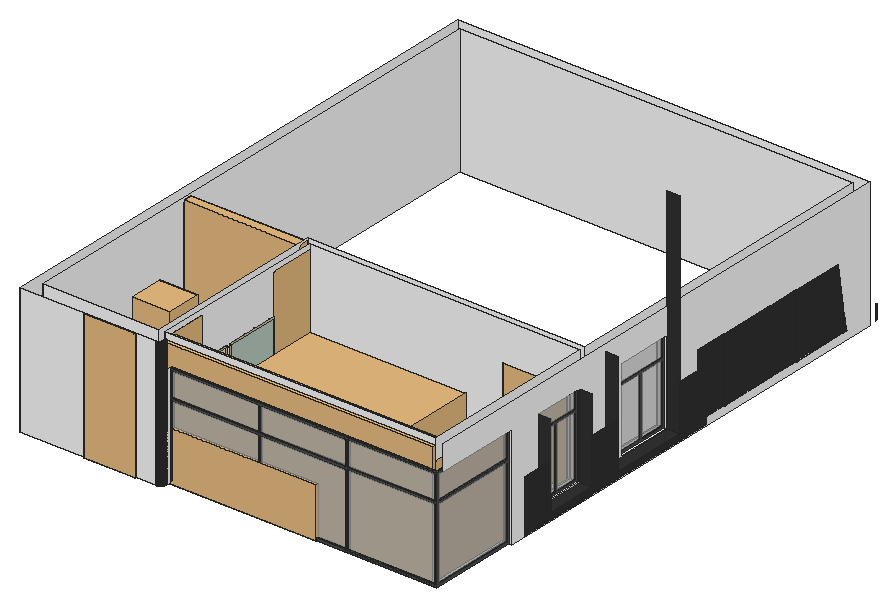
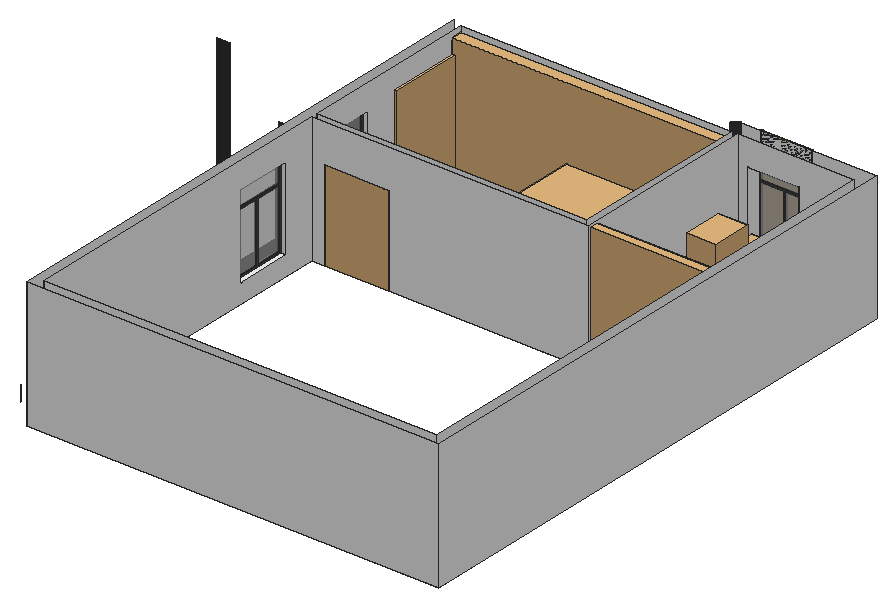
# SketchUp Ruby script. Lengths in inches.
U = 1.inch
M = Sketchup.active_model
def pt(a) = Geom::Point3d.new(a.map { |v| v * U })
def face(e, loops, mat)
  f = e.add_face(loops[0].map { |a| pt(a) })
  loops[1..].each { |l| e.add_face(l.map { |a| pt(a) }).erase! }
  f.material = f.back_material = mat if mat
  f
end
# faces: each face lists its corners as indices into pts; further lists are holes
def faces(e, pts, list, mat = nil) = list.each { |f| face(e, (f[0].is_a?(Array) ? f : [f]).map { |l| l.map { |i| pts[i] } }, mat) }
# xy, xz, yz: faces in a plane at the given z, y or x. An outline is a flat list of corners, or four numbers for a rectangle; further outlines are holes
def ring(l) = l.size == 4 ? [[l[0], l[1]], [l[2], l[1]], [l[2], l[3]], [l[0], l[3]]] : l.each_slice(2).to_a
def flat(e, list, mat, &to3) = list.each { |f| face(e, (f[0].is_a?(Array) ? f : [f]).map { |l| ring(l).map { |u, v| to3.(u, v) } }, mat) }
def xy(e, z, list, mat = nil) = flat(e, list, mat) { |x, y| [x, y, z] }
def xz(e, y, list, mat = nil) = flat(e, list, mat) { |x, z| [x, y, z] }
def yz(e, x, list, mat = nil) = flat(e, list, mat) { |y, z| [x, y, z] }
def lines(e, pts, list) = list.each { |a, b| e.add_line(pt(pts[a]), pt(pts[b])) }
# prism: a flat outline (further loops are holes) pulled along v
def prism(e, loops, v, mat = nil)
  f = face(e, loops, mat); d = Geom::Vector3d.new(v.map { |x| x * U })
  f.pushpull(f.normal.samedirection?(d) ? d.length : -d.length)
end
def box(e, o, s, mat = nil) = prism(e, [[o, [o[0] + s[0], o[1], o[2]], [o[0] + s[0], o[1] + s[1], o[2]], [o[0], o[1] + s[1], o[2]]]], [0, 0, s[2]], mat)
def at(x, y, z, deg = 0) = Geom::Transformation.translation(pt([x, y, z])) * Geom::Transformation.rotation(ORIGIN, Z_AXIS, deg.degrees)
def axes(o, x, y, z) = Geom::Transformation.new([*x, 0, *y, 0, *z, 0, *pt(o).to_a, 1])
def part(name) = M.definitions.add(name)
# library, detail: a bought-in or finely detailed component or shape, given as its bounding box
def library(name, o, s) = part(name).tap { |d| box(d.entities, o, s) }
def detail(e, o, s) = box(e.add_group.entities, o, s)
def put(e, d, t, mat = nil) = e.add_instance(d, t).tap { |i| i.material = mat if mat }
def group(e, t, mat = nil) = e.add_group.tap { |g| g.transformation = t; g.material = mat if mat }.entities
root = M.entities
M.materials.add("12_plywood texture-seamless").color = [215, 194, 159]
M.materials.add("[Color_001]2").color = [144, 137, 126]
M.materials.add("[Color_005]1").color = [178, 182, 175]
M.materials.add("[Granite Dark Gray]").color = [51, 50, 50]
M.materials.add("[Metal Seamed]").color = [79, 80, 77]
M.materials.add("[Quartz Light Grey]").color = [251, 251, 252]
M.materials.add("[Translucent Glass Gray]").color = [183, 183, 183]
M.materials["[Translucent Glass Gray]"].alpha = 0.5
M.materials.add("[Wood Veneer 01]1").color = [120, 70, 37]
M.materials.add("il_570xN.1307621332_kpxq").color = [189, 207, 195]
M.materials.add("il_570xN.1571116333_4k0l").color = [234, 234, 226]
c1 = library("plant\#1",[-21.34,-27.21,-0.38],[41.91,41.15,38.97])
c2 = library("Classic grayblue sofa  living room ",[-100.93,-81.02,-0.06],[174.43,145.32,46.54])
c3 = library("small sofa",[87.94,-13.34,0],[66.53,49.05,32.95])
c4 = part("6\#1")
g1 = group(c4.entities,at(25.4,42.84,0),"[Color_001]2")
box(g1,[0,0,0],[104,190.3125,0.89],"[Color_005]1")
c5 = library("Plante 4",[-1.67,-6.5,0],[37.31,31.95,64.42])
c6 = library("Group\#15",[0,-0.5,0],[48,0.5,120])
c7 = part("Group\#22")
box(c7.entities,[0,-0.47,69],[80.67,0.47,23])
box(c7.entities,[0,-0.47,0],[80.67,0.47,67])
c8 = library("Group\#62",[0,0,0],[0.25,42,120])
c9 = library("Group\#68",[0,0,0],[0.25,42,120])
c10 = library("SLIDING+GLASS+DOOR",[0,-0.75,0],[72,5.75,80])
c11 = library("Curtains and rod",[2.63,-1.46,0.02],[153.32,14.02,114.15])
c12 = library("Curtains",[0,0,0],[121.73,8.19,117.22])
c13 = library("---------1\#1",[5.49,6.625,-77.21],[69.81,13.39,114.05])
c14 = part("Agrupar\#2")
xy(c14.entities,0,[[0,0,15.75,21.65]])
xy(c14.entities,0.59,[[0,0,15.75,21.65]],"il_570xN.1571116333_4k0l")
xz(c14.entities,0,[[0,0,15.75,0.59]])
xz(c14.entities,21.65,[[0,0,15.75,0.59]])
yz(c14.entities,0,[[0,0,21.65,0.59]])
yz(c14.entities,15.75,[[0,0,21.65,0.59]])
c15 = part("Agrupar\#4")
xy(c15.entities,0,[[[0.3,0.3,17.03,22.93],[0.79,0.79,16.54,22.44]]],"12_plywood texture-seamless")
xy(c15.entities,0.79,[[0.3,0.3,0.79,0.79,0.79,22.44,0.3,22.93],[0.3,0.3,17.03,0.3,16.54,0.79,0.79,0.79],[17.03,0.3,17.03,22.93,16.54,22.44,16.54,0.79],[0.79,22.44,16.54,22.44,17.03,22.93,0.3,22.93]],"12_plywood texture-seamless")
xz(c15.entities,0.3,[[0.3,0,17.03,0.79]],"12_plywood texture-seamless")
xz(c15.entities,0.79,[[0.79,0,16.54,0.79]],"12_plywood texture-seamless")
xz(c15.entities,22.44,[[0.79,0,16.54,0.79]],"12_plywood texture-seamless")
xz(c15.entities,22.93,[[0.3,0,17.03,0.79]],"12_plywood texture-seamless")
yz(c15.entities,0.3,[[0.3,0,22.93,0.79]],"12_plywood texture-seamless")
yz(c15.entities,0.79,[[0.79,0,22.44,0.79]],"12_plywood texture-seamless")
yz(c15.entities,16.54,[[0.79,0,22.44,0.79]],"12_plywood texture-seamless")
yz(c15.entities,17.03,[[0.3,0,22.93,0.79]],"12_plywood texture-seamless")
c16 = part("Agrupar\#1")
put(c16.entities,c14,at(0.79,0.79,0))
put(c16.entities,c15,at(0,0,0))
c17 = part("Agrupar\#3")
xy(c17.entities,0,[[-3.44,0,15.75,26.08]])
xy(c17.entities,0.59,[[-3.44,0,15.75,26.08]],"il_570xN.1307621332_kpxq")
xz(c17.entities,0,[[-3.44,0,15.75,0.59]])
xz(c17.entities,26.08,[[-3.44,0,15.75,0.59]])
yz(c17.entities,-3.44,[[0,0,26.08,0.59]])
yz(c17.entities,15.75,[[0,0,26.08,0.59]])
c18 = part("Agrupar\#7")
xy(c18.entities,0,[[[-3.15,0.3,17.03,27.36],[-2.66,0.79,16.54,26.87]]],"12_plywood texture-seamless")
xy(c18.entities,0.79,[[-3.15,0.3,-3.15,27.36,-2.66,26.87,-2.66,0.79],[-3.15,0.3,17.03,0.3,16.54,0.79,-2.66,0.79],[17.03,0.3,16.54,0.79,16.54,26.87,17.03,27.36],[-2.66,26.87,-3.15,27.36,17.03,27.36,16.54,26.87]],"12_plywood texture-seamless")
xz(c18.entities,0.3,[[-3.15,0,17.03,0.79]],"12_plywood texture-seamless")
xz(c18.entities,0.79,[[-2.66,0,16.54,0.79]],"12_plywood texture-seamless")
xz(c18.entities,26.87,[[-2.66,0,16.54,0.79]],"12_plywood texture-seamless")
xz(c18.entities,27.36,[[-3.15,0,17.03,0.79]],"12_plywood texture-seamless")
yz(c18.entities,-3.15,[[0.3,0,27.36,0.79]],"12_plywood texture-seamless")
yz(c18.entities,-2.66,[[0.79,0,26.87,0.79]],"12_plywood texture-seamless")
yz(c18.entities,16.54,[[0.79,0,26.87,0.79]],"12_plywood texture-seamless")
yz(c18.entities,17.03,[[0.3,0,27.36,0.79]],"12_plywood texture-seamless")
c19 = part("Agrupar\#8")
put(c19.entities,c17,at(0.79,0.79,0))
put(c19.entities,c18,at(0,0,0))
c20 = part("CALIFORNIA WALL ART")
put(c20.entities,c16,axes([-38.21,13.68,-7.42],[0.78256,0,0],[0,0,0.78256],[0,-0.78256,0]))
put(c20.entities,c19,axes([-23.17,13.75,7.77],[0,0,-0.878],[0.878,0,0],[0,-0.878,0]))
xy(root,138,[[48,90,48,600,432,600,432,183,423,183,423,591,57,591,57,105,165,105,165,279,351,279,351,273,171,273,171,105,180,105,180,95.78,179.95,95.23,179.93,95.12,179.92,95.01,179.9,94.9,179.85,94.68,179.83,94.57,179.8,94.46,179.77,94.36,179.74,94.25,179.71,94.15,179.67,94.04,179.63,93.9375,179.59,93.83,179.47,93.53,179.27,93.13,179.21,93.03,179.16,92.9375,179.1,92.84,178.98,92.66,178.92,92.5625,178.85,92.47,178.79,92.38,178.72,92.3,178.65,92.21,178.51,92.04,178.43,91.96,178.36,91.875,178.28,91.8,178.2,91.72,178.125,91.64,178.04,91.57,177.96,91.49,177.79,91.35,177.7,91.28,177.62,91.21,177.53,91.15,177.4375,91.08,177.34,91.02,177.16,90.9,177.0625,90.84,176.97,90.79,176.87,90.73,176.47,90.53,176.17,90.41,176.0625,90.37,175.96,90.33,175.85,90.29,175.75,90.26,175.64,90.23,175.54,90.2,175.43,90.17,175.32,90.15,175.1,90.1,174.99,90.08,174.88,90.07,174.77,90.05,174.22,90],[411,273,423,279]],"[Quartz Light Grey]")
xy(root,150,[[443.875,183,444,207],[443.875,208,444,213],[443.875,213,444,261],[443.875,261,444,267],[443.875,268,444,291],
  [443.875,291,444,303],[443.875,304,444,369],[443.875,370,444,393],[436.875,393,437,423],[436.875,424,437,477],
  [436.875,478,437,507],[436.875,508,437,562],[436.875,563,437,565.83]],"[Granite Dark Gray]")
xy(root,151,[[443.875,183,444,207],[443.875,208,444,213],[443.875,213,444,261],[443.875,261,444,267],[443.875,268,444,291],
  [443.875,291,444,369],[443.875,370,444,393],[436.875,393,437,423],[436.875,424,437,477],[436.875,478,437,507],
  [436.875,508,437,562],[436.875,563,437,565.65]],"[Granite Dark Gray]")
xy(root,156,[[432,213,444,261],[432,291,444,363]],"[Granite Dark Gray]")
xy(root,156,[[423,213,432,261],[423,309,432,363]],"[Quartz Light Grey]")
xy(root,162,[[108,90,156,105]],"[Quartz Light Grey]")
xz(root,90,[[[48,138,174,258],[108,162,156,234]],[174,138,174.11,258],[174.11,138,174.22,258]],"[Quartz Light Grey]")
xz(root,105,[[[57,138,165,258],[108,162,156,234]],[171,138,171,258,423,258,423,234,180,234,180,138]],"[Quartz Light Grey]")
xz(root,183,[[423,138,432,234]],"[Quartz Light Grey]")
xz(root,207,[[443.875,151,444,199]],"[Granite Dark Gray]")
xz(root,208,[[443.875,151,444,199]],"[Granite Dark Gray]")
xz(root,213,[[432,156,432,234,444,234,444,200,443.875,200,443.875,199,444,199,444,156]],"[Granite Dark Gray]")
xz(root,213,[[423,156,432,234]],"[Quartz Light Grey]")
xz(root,261,[[432,156,444,156,444,199,443.875,199,443.875,200,444,200,444,234,432,234]],"[Granite Dark Gray]")
xz(root,261,[[423,156,432,234]],"[Quartz Light Grey]")
xz(root,267,[[443.875,151,444,199]],"[Granite Dark Gray]")
xz(root,268,[[443.875,151,444,199]],"[Granite Dark Gray]")
xz(root,273,[[171,138,351,138,351,222,411,222,411,138,423,138,423,258,171,258]],"[Quartz Light Grey]")
xz(root,279,[[165,138,165,258,423,258,423,138,411,138,411,222,351,222,351,138]],"[Quartz Light Grey]")
xz(root,291,[[432,156,432,252,444,252,444,249,443.875,249,443.875,248,444,248,444,200,443.875,200,443.875,199,444,199,444,156]],"[Granite Dark Gray]")
xz(root,309,[[423,156,432,234]],"[Quartz Light Grey]")
xz(root,363,[[432,156,444,156,444,199,443.875,199,443.875,200,444,200,444,248,443.875,248,443.875,249,444,249,444,278,443.875,278,443.875,279,444,279,444,332,443.875,332,443.875,333,444,333,444,354,432,354]],"[Granite Dark Gray]")
xz(root,363,[[423,156,432,234]],"[Quartz Light Grey]")
xz(root,369,[[443.875,151,444,199]],"[Granite Dark Gray]")
xz(root,370,[[443.875,151,444,199]],"[Granite Dark Gray]")
xz(root,423,[[436.875,151,437,210]],"[Granite Dark Gray]")
xz(root,424,[[436.875,151,437,210]],"[Granite Dark Gray]")
xz(root,477,[[436.875,151,437,210]],"[Granite Dark Gray]")
xz(root,478,[[436.875,151,437,210]],"[Granite Dark Gray]")
xz(root,507,[[436.875,151,437,210]],"[Granite Dark Gray]")
xz(root,508,[[436.875,151,437,210]],"[Granite Dark Gray]")
xz(root,562,[[436.875,151,437,172]],"[Granite Dark Gray]")
xz(root,563,[[436.875,151,437,166.25]],"[Granite Dark Gray]")
xz(root,591,[[443.875,150,444,151],[443.875,151,444,164]],"[Granite Dark Gray]")
xz(root,591,[[57,138,423,258]],"[Quartz Light Grey]")
xz(root,592,[[443.875,150,444,151],[443.875,151,444,164]],"[Granite Dark Gray]")
xz(root,600,[[48,138,432,258]],"[Quartz Light Grey]")
yz(root,48,[[90,138,600,258]],"[Quartz Light Grey]")
yz(root,57,[[105,138,591,258]],"[Quartz Light Grey]")
yz(root,108,[[90,162,105,234]],"[Quartz Light Grey]")
yz(root,156,[[90,162,105,234]],"[Quartz Light Grey]")
yz(root,165,[[105,138,279,258]],"[Quartz Light Grey]")
yz(root,171,[[105,138,273,258]],"[Quartz Light Grey]")
yz(root,180,[[95.78,138,95.89,258],[95.89,138,96,258],[96,138,105,234]],"[Quartz Light Grey]")
yz(root,351,[[273,138,279,222]],"[Quartz Light Grey]")
yz(root,411,[[273,138,279,222]],"[Quartz Light Grey]")
yz(root,423,[[[183,138,183,234,105,234,105,258,273,258,273,138],[213,156,261,234]],[[279,138,591,258],[309,156,363,234]]],"[Quartz Light Grey]")
yz(root,432,[[[183,138,600,138,600,258,102,258,102,234,183,234],[309,156,363,234],[213,156,261,234]]],"[Quartz Light Grey]")
yz(root,437,[[393,151,423,210],[424,151,477,210],[478,151,507,210],[508,151,562,151,562,172,555.39,210,508,210],[563,151,565.65,151,563,166.25]],"[Granite Dark Gray]")
yz(root,444,[[183,151,207,199],[208,151,267,151,267,199,261,199,261,156,213,156,213,199,208,199],[268,151,369,151,369,199,363,199,363,156,291,156,291,199,268,199],[370,151,393,199]],"[Granite Dark Gray]")
p = [[174.22,90,138],[174.33,90.01,138],[174.33,90.01,258],[174.22,90,258],[174.44,90.02,138],[174.44,90.02,258],
  [174.55,90.03,138],[174.55,90.03,258],[174.66,90.04,138],[174.66,90.04,258],[174.77,90.05,138],[174.77,90.05,258],
  [174.88,90.07,138],[174.88,90.07,258],[174.99,90.08,138],[174.99,90.08,258],[175.1,90.1,138],[175.1,90.1,258],
  [175.21,90.125,138],[175.21,90.125,258],[175.32,90.15,138],[175.32,90.15,258],[175.43,90.17,138],[175.43,90.17,258],
  [175.54,90.2,138],[175.54,90.2,258],[175.64,90.23,138],[175.64,90.23,258],[175.75,90.26,138],[175.75,90.26,258],
  [175.85,90.29,138],[175.85,90.29,258],[175.96,90.33,138],[175.96,90.33,258],[176.0625,90.37,138],[176.0625,90.37,258],
  [176.17,90.41,138],[176.17,90.41,258],[176.27,90.45,138],[176.27,90.45,258],[176.37,90.49,138],[176.37,90.49,258],
  [176.47,90.53,138],[176.47,90.53,258],[176.57,90.58,138],[176.57,90.58,258],[176.67,90.63,138],[176.67,90.63,258],
  [176.77,90.68,138],[176.77,90.68,258],[176.87,90.73,138],[176.87,90.73,258],[176.97,90.79,138],[176.97,90.79,258],
  [177.0625,90.84,138],[177.0625,90.84,258],[177.16,90.9,138],[177.16,90.9,258],[177.25,90.96,138],[177.25,90.96,258],
  [177.34,91.02,138],[177.4375,91.08,138],[177.4375,91.08,258],[177.34,91.02,258],[177.53,91.15,138],[177.53,91.15,258],
  [177.62,91.21,138],[177.62,91.21,258],[177.7,91.28,138],[177.7,91.28,258],[177.79,91.35,138],[177.79,91.35,258],
  [177.875,91.42,138],[177.875,91.42,258],[177.96,91.49,138],[177.96,91.49,258],[178.04,91.57,138],[178.04,91.57,258],
  [178.125,91.64,138],[178.125,91.64,258],[178.2,91.72,138],[178.2,91.72,258],[178.28,91.8,138],[178.28,91.8,258],
  [178.36,91.875,138],[178.36,91.875,258],[178.43,91.96,138],[178.43,91.96,258],[178.51,92.04,138],[178.51,92.04,258],
  [178.58,92.125,138],[178.58,92.125,258],[178.65,92.21,138],[178.65,92.21,258],[178.72,92.3,138],[178.72,92.3,258],
  [178.79,92.38,138],[178.79,92.38,258],[178.85,92.47,138],[178.85,92.47,258],[178.92,92.5625,138],[178.92,92.5625,258],
  [178.98,92.66,138],[178.98,92.66,258],[179.04,92.75,138],[179.1,92.84,138],[179.1,92.84,258],[179.04,92.75,258],
  [179.16,92.9375,138],[179.16,92.9375,258],[179.21,93.03,138],[179.21,93.03,258],[179.27,93.13,138],[179.27,93.13,258],
  [179.32,93.23,138],[179.32,93.23,258],[179.37,93.33,138],[179.37,93.33,258],[179.42,93.43,138],[179.42,93.43,258],
  [179.47,93.53,138],[179.47,93.53,258],[179.51,93.63,138],[179.51,93.63,258],[179.55,93.73,138],[179.55,93.73,258],
  [179.59,93.83,138],[179.59,93.83,258],[179.63,93.9375,138],[179.63,93.9375,258],[179.67,94.04,138],[179.67,94.04,258],
  [179.71,94.15,138],[179.71,94.15,258],[179.74,94.25,138],[179.74,94.25,258],[179.77,94.36,138],[179.77,94.36,258],
  [179.8,94.46,138],[179.8,94.46,258],[179.83,94.57,138],[179.83,94.57,258],[179.85,94.68,138],[179.85,94.68,258],
  [179.875,94.79,138],[179.875,94.79,258],[179.9,94.9,138],[179.9,94.9,258],[179.92,95.01,138],[179.92,95.01,258],
  [179.93,95.12,138],[179.93,95.12,258],[179.95,95.23,138],[179.95,95.23,258],[179.96,95.34,138],[179.96,95.34,258],
  [179.97,95.45,138],[179.97,95.45,258],[179.98,95.56,138],[179.98,95.56,258],[179.99,95.67,138],[179.99,95.67,258],
  [180,95.78,138],[180,95.78,258],[437,565.65,151],[437,565.83,151]]
faces(root,p,[[0,1,2,3],[1,4,5,2],[4,6,7,5],[6,8,9,7],[8,10,11,9],[10,12,13,11],[12,14,15,13],[14,16,17,15],
  [16,18,19,17],[18,20,21,19],[20,22,23,21],[22,24,25,23],[24,26,27,25],[26,28,29,27],[28,30,31,29],[30,32,33,31],
  [32,34,35,33],[34,36,37,35],[36,38,39,37],[38,40,41,39],[40,42,43,41],[42,44,45,43],[44,46,47,45],[46,48,49,47],
  [48,50,51,49],[50,52,53,51],[52,54,55,53],[54,56,57,55],[56,58,59,57],[60,61,62,63],[58,60,63,59],[61,64,65,62],
  [64,66,67,65],[66,68,69,67],[68,70,71,69],[70,72,73,71],[72,74,75,73],[74,76,77,75],[76,78,79,77],[78,80,81,79],
  [80,82,83,81],[82,84,85,83],[84,86,87,85],[86,88,89,87],[88,90,91,89],[90,92,93,91],[92,94,95,93],[94,96,97,95],
  [96,98,99,97],[98,100,101,99],[100,102,103,101],[104,105,106,107],[102,104,107,103],[105,108,109,106],[108,110,111,109],[110,112,113,111],
  [112,114,115,113],[114,116,117,115],[116,118,119,117],[118,120,121,119],[120,122,123,121],[122,124,125,123],[124,126,127,125],[126,128,129,127],
  [128,130,131,129],[130,132,133,131],[132,134,135,133],[134,136,137,135],[136,138,139,137],[138,140,141,139],[140,142,143,141],[142,144,145,143],
  [144,146,147,145],[146,148,149,147],[148,150,151,149],[150,152,153,151],[152,154,155,153],[154,156,157,155],[156,158,159,157],[158,160,161,159],
  [160,162,163,161]],"[Quartz Light Grey]")
lines(root,p,[[164,165]])
put(root,c1,at(153.01,128.4,138),"[Quartz Light Grey]")
put(root,c2,at(235.55,199.5,138.06,90),"[Quartz Light Grey]")
put(root,c3,at(-30.94,181.03,138),"[Quartz Light Grey]")
put(root,c4,axes([53.26,104.99,138],[0.57372,0,0],[0,0.47,0],[0,0,0.47]),"[Quartz Light Grey]")
put(root,c5,at(57.61,214.58,138),"[Quartz Light Grey]")
put(root,c5,at(143.02,164.16,138,-90),"[Quartz Light Grey]")
put(root,c6,at(108,90,138),"[Wood Veneer 01]1")
g2 = group(root,at(180,99,138),"[Quartz Light Grey]")
xy(g2,0,[[0,0,0,2,247,2,247,84,249,84,249,0]],"[Metal Seamed]")
xy(g2,2,[[2,0,82.67,2],[84.67,0,164.33,2],[166.33,0,247,2],[247,2,249,82]],"[Metal Seamed]")
xy(g2,69,[[2,0,82.67,2],[84.67,0,164.33,2],[166.33,0,247,2],[247,2,249,82]],"[Metal Seamed]")
xy(g2,71,[[2,0,82.67,2],[84.67,0,164.33,2],[166.33,0,247,2],[247,2,249,82]],"[Metal Seamed]")
xy(g2,94,[[2,0,82.67,2],[84.67,0,164.33,2],[166.33,0,247,2],[247,2,249,82]],"[Metal Seamed]")
xy(g2,96,[[0,0,249,0,249,84,247,84,247,2,0,2]],"[Metal Seamed]")
xz(g2,0,[[[0,0,249,96],[166.33,2,247,69],[2,2,82.67,69],[84.67,2,164.33,69],[2,71,82.67,94],[166.33,71,247,94],[84.67,71,164.33,94]]],"[Metal Seamed]")
xz(g2,2,[[[0,0,0,96,247,96,247,94,166.33,94,166.33,71,247,71,247,69,166.33,69,166.33,2,247,2,247,0],[2,2,82.67,69],[84.67,2,164.33,69],[2,71,82.67,94],[84.67,71,164.33,94]],[247,2,249,69],[247,71,249,94]],"[Metal Seamed]")
xz(g2,82,[[247,2,249,69],[247,71,249,94]],"[Metal Seamed]")
xz(g2,84,[[247,0,249,96]],"[Metal Seamed]")
yz(g2,0,[[0,0,2,96]],"[Metal Seamed]")
yz(g2,2,[[0,2,2,69],[0,71,2,94]],"[Metal Seamed]")
yz(g2,82.67,[[0,2,2,69],[0,71,2,94]],"[Metal Seamed]")
yz(g2,84.67,[[0,2,2,69],[0,71,2,94]],"[Metal Seamed]")
yz(g2,164.33,[[0,2,2,69],[0,71,2,94]],"[Metal Seamed]")
yz(g2,166.33,[[0,2,2,69],[0,71,2,94]],"[Metal Seamed]")
yz(g2,247,[[2,0,2,2,82,2,82,69,2,69,2,71,82,71,82,94,2,94,2,96,84,96,84,0],[0,2,2,69],[0,71,2,94]],"[Metal Seamed]")
yz(g2,249,[[[0,0,84,96],[2,2,82,69],[2,71,82,94]]],"[Metal Seamed]")
put(g2,c7,at(2,1.25,2),"[Translucent Glass Gray]")
put(g2,c7,axes([84.67,1.25,2],[0.9876,0,0],[0,1,0],[0,0,1]),"[Translucent Glass Gray]")
put(g2,c7,at(166.33,1.25,2),"[Translucent Glass Gray]")
put(g2,c7,axes([247.75,2,2],[0,0.99174,0],[-1,0,0],[0,0,1]),"[Translucent Glass Gray]")
put(root,c8,axes([171,231,138],[1,0,0],[0,1,0],[0,0,0.96]),"[Quartz Light Grey]")
put(root,c9,axes([171,105,138],[1,0,0],[0,1,0],[0,0,0.96]),"[Quartz Light Grey]")
put(root,c10,axes([351,274,138],[0.83333,0,0],[0,1,0],[0,0,1.05]),"[Quartz Light Grey]")
put(root,c11,axes([166.67,102.76,138.27],[1.64362,0,0],[0,1,0],[0,0,1]),"[Quartz Light Grey]")
put(root,c12,axes([57,269.45,138.9375],[0.88723,0,0],[0,1,0],[0,0,1]))
put(root,c13,axes([418.6,98.86,206.76],[0,1.11742,0],[0.22,0,0],[0,0,0.87516]),"[Quartz Light Grey]")
g3 = group(root,at(428,309,156),"[Quartz Light Grey]")
p = [[0,52.5,1.5],[0,52.5,57],[0,52.5,76.5],[0,1.5,76.5],[0,1.5,58.5],[0,1.5,1.5],
  [0,26.25,1.5],[0,52.5,58.5],[0,27.75,57],[0,1.5,57],[0,26.25,57],[0,27.75,1.5]]
lines(g3,p,[[0,1],[2,3],[3,4],[5,6],[7,4],[7,2],[1,8],[9,5],[10,6],[10,9],[8,11],[11,0]])
g4 = group(g3,at(0,0,0),"[Metal Seamed]")
prism(g4,[[[0,54,78],[0,54,0],[0,0,0],[0,0,78]],[[0,26.25,1.5],[0,26.25,57],[0,1.5,57],[0,1.5,1.5]],[[0,27.75,1.5],[0,52.5,1.5],[0,52.5,57],[0,27.75,57]],[[0,52.5,58.5],[0,52.5,76.5],[0,1.5,76.5],[0,1.5,58.5]]],[1.5,0,0])
g5 = group(g4,at(0.5,1.5,1.5))
box(g5,[0,26.25,0],[0.47,24.75,55.5],"[Translucent Glass Gray]")
box(g5,[0,0,0],[0.47,24.75,55.5],"[Translucent Glass Gray]")
box(g5,[0,0,57],[0.47,51,18],"[Translucent Glass Gray]")
g6 = group(root,at(428.5,213,156),"[Quartz Light Grey]")
p = [[0,1.5,76.5],[0,1.5,60.5],[0,1.5,1.5],[0,23.25,1.5],[0,46.5,1.5],[0,46.5,59],
  [0,46.5,76.5],[0,46.5,60.5],[0,24.75,59],[0,1.5,59],[0,23.25,59],[0,24.75,1.5]]
lines(g6,p,[[0,1],[2,3],[4,5],[6,0],[7,1],[7,6],[5,8],[9,2],[10,3],[10,9],[8,11],[11,4]])
g7 = group(g6,at(0,0,0))
prism(g7,[[[0,48,78],[0,48,0],[0,0,0],[0,0,78]],[[0,23.25,1.5],[0,23.25,59],[0,1.5,59],[0,1.5,1.5]],[[0,24.75,1.5],[0,46.5,1.5],[0,46.5,59],[0,24.75,59]],[[0,46.5,60.5],[0,46.5,76.5],[0,1.5,76.5],[0,1.5,60.5]]],[1.5,0,0],"[Metal Seamed]")
g8 = group(g7,at(0.5,1.5,1.5),"[Translucent Glass Gray]")
box(g8,[0,0,59],[0.47,45,16])
box(g8,[0,23.25,0],[0.47,21.75,57.5])
box(g8,[0,0,0],[0.47,21.75,57.5])
put(root,c20,axes([184.75,229.16,183.9],[0,2.16343,0],[-1,0,0],[0,0,3.04817]),"[Quartz Light Grey]")
g9 = group(root,at(108,92,162),"[Quartz Light Grey]")
p = [[46.5,0,1.5],[46.5,0,54],[46.5,0,70.5],[1.5,0,70.5],[1.5,0,55.5],[1.5,0,1.5],
  [23.25,0,1.5],[46.5,0,55.5],[24.75,0,54],[1.5,0,54],[23.25,0,54],[24.75,0,1.5]]
lines(g9,p,[[0,1],[2,3],[3,4],[5,6],[7,4],[7,2],[1,8],[9,5],[10,6],[10,9],[8,11],[11,0]])
g10 = group(g9,at(0,0,0),"[Metal Seamed]")
prism(g10,[[[0,0,72],[48,0,72],[48,0,0],[0,0,0]],[[24.75,0,1.5],[46.5,0,1.5],[46.5,0,54],[24.75,0,54]],[[23.25,0,1.5],[23.25,0,54],[1.5,0,54],[1.5,0,1.5]],[[46.5,0,55.5],[46.5,0,70.5],[1.5,0,70.5],[1.5,0,55.5]]],[0,-1.5,0])
g11 = group(g10,at(1.5,-0.5,1.5))
box(g11,[0,-0.47,0],[21.75,0.47,52.5],"[Translucent Glass Gray]")
box(g11,[0,-0.47,54],[45,0.47,15],"[Translucent Glass Gray]")
box(g11,[23.25,-0.47,0],[21.75,0.47,52.5],"[Translucent Glass Gray]")
